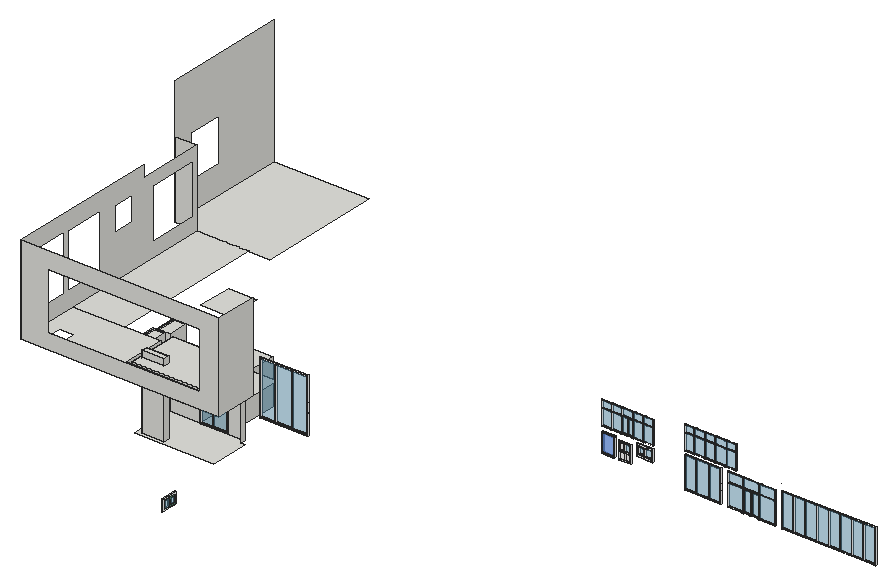
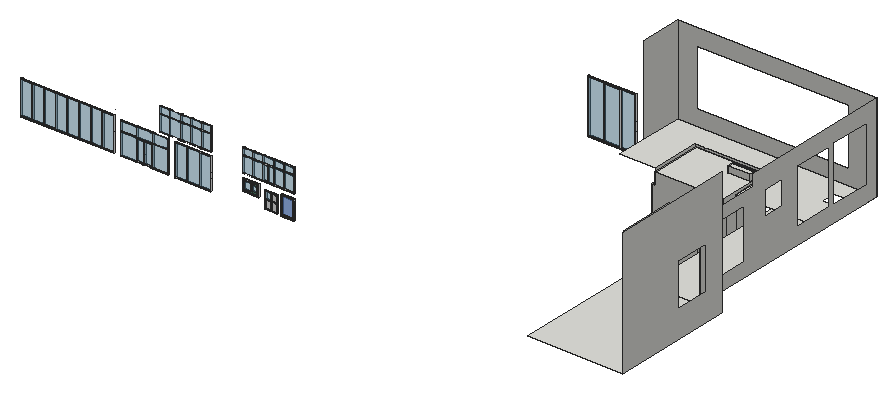
# SketchUp Ruby script. Lengths in inches.
U = 1.inch
M = Sketchup.active_model
def pt(a) = Geom::Point3d.new(a.map { |v| v * U })
def face(e, loops, mat)
  f = e.add_face(loops[0].map { |a| pt(a) })
  loops[1..].each { |l| e.add_face(l.map { |a| pt(a) }).erase! }
  f.material = f.back_material = mat if mat
  f
end
# faces: each face lists its corners as indices into pts; further lists are holes
def faces(e, pts, list, mat = nil) = list.each { |f| face(e, (f[0].is_a?(Array) ? f : [f]).map { |l| l.map { |i| pts[i] } }, mat) }
# xy, xz, yz: faces in a plane at the given z, y or x. An outline is a flat list of corners, or four numbers for a rectangle; further outlines are holes
def ring(l) = l.size == 4 ? [[l[0], l[1]], [l[2], l[1]], [l[2], l[3]], [l[0], l[3]]] : l.each_slice(2).to_a
def flat(e, list, mat, &to3) = list.each { |f| face(e, (f[0].is_a?(Array) ? f : [f]).map { |l| ring(l).map { |u, v| to3.(u, v) } }, mat) }
def xy(e, z, list, mat = nil) = flat(e, list, mat) { |x, y| [x, y, z] }
def xz(e, y, list, mat = nil) = flat(e, list, mat) { |x, z| [x, y, z] }
def yz(e, x, list, mat = nil) = flat(e, list, mat) { |y, z| [x, y, z] }
def lines(e, pts, list) = list.each { |a, b| e.add_line(pt(pts[a]), pt(pts[b])) }
# prism: a flat outline (further loops are holes) pulled along v
def prism(e, loops, v, mat = nil)
  f = face(e, loops, mat); d = Geom::Vector3d.new(v.map { |x| x * U })
  f.pushpull(f.normal.samedirection?(d) ? d.length : -d.length)
end
def box(e, o, s, mat = nil) = prism(e, [[o, [o[0] + s[0], o[1], o[2]], [o[0] + s[0], o[1] + s[1], o[2]], [o[0], o[1] + s[1], o[2]]]], [0, 0, s[2]], mat)
def at(x, y, z, deg = 0) = Geom::Transformation.translation(pt([x, y, z])) * Geom::Transformation.rotation(ORIGIN, Z_AXIS, deg.degrees)
def axes(o, x, y, z) = Geom::Transformation.new([*x, 0, *y, 0, *z, 0, *pt(o).to_a, 1])
def part(name) = M.definitions.add(name)
# library, detail: a bought-in or finely detailed component or shape, given as its bounding box
def library(name, o, s) = part(name).tap { |d| box(d.entities, o, s) }
def detail(e, o, s) = box(e.add_group.entities, o, s)
def put(e, d, t, mat = nil) = e.add_instance(d, t).tap { |i| i.material = mat if mat }
def group(e, t, mat = nil) = e.add_group.tap { |g| g.transformation = t; g.material = mat if mat }.entities
root = M.entities
M.materials.add("Translucent_Glass_Blue1").color = [100, 149, 237]
M.materials["Translucent_Glass_Blue1"].alpha = 0.5
M.materials.add("[0010_Snow]").color = [255, 250, 250]
M.materials.add("[Color_000]").color = [255, 255, 255]
M.materials.add("[Jade]").color = [77, 143, 110]
M.materials.add("[Translucent_Glass_Blue]").color = [100, 149, 237]
M.materials["[Translucent_Glass_Blue]"].alpha = 0.5
M.materials.add("[Translucent_Glass_Blue]1").color = [87, 149, 181]
M.materials["[Translucent_Glass_Blue]1"].alpha = 0.5
c1 = part("Group\#3")
xy(c1.entities,0,[[0,0,2.14,2.21]],"[Color_000]")
xy(c1.entities,1.67,[[2.14,0,29.96,2.21],[29.96,0,32.1,0.88],[32.1,0,64.19,2.21],[64.19,0,66.33,0.88]],"[Color_000]")
xy(c1.entities,84.95,[[2.14,0,29.96,2.21],[29.96,0,32.1,0.88],[32.1,0,64.19,2.21],[64.19,0,66.33,0.88]],"[Color_000]")
xy(c1.entities,86.61,[[0,0,66.33,2.21]],"[Color_000]")
xz(c1.entities,0,[[0,0,0,86.61,66.33,86.61,66.33,84.95,2.14,84.95,2.14,0],[2.14,0,66.33,1.67]],"[Color_000]")
xz(c1.entities,0.88,[[29.96,1.67,32.1,84.95],[64.19,1.67,66.33,84.95]],"[Color_000]")
xz(c1.entities,2.21,[[2.14,1.67,29.96,84.95],[32.1,1.67,64.19,84.95]],"[Translucent_Glass_Blue]1")
yz(c1.entities,0,[[0,0,2.21,32.8125],[0,32.8125,2.21,48.3],[0,48.3,2.21,86.61]],"[Color_000]")
yz(c1.entities,2.14,[[0,1.67,2.21,84.95]],"[Color_000]")
yz(c1.entities,29.96,[[0.88,1.67,2.21,84.95]],"[Color_000]")
yz(c1.entities,32.1,[[0.88,1.67,2.21,84.95]],"[Color_000]")
yz(c1.entities,64.19,[[0.88,1.67,2.21,84.95]],"[Color_000]")
yz(c1.entities,66.33,[[0.88,1.67,2.21,84.95]],"[Color_000]")
c2 = part("ProLine-Casement-Window")
xy(c2.entities,-3.73,[[[0,0,29,59],[0.74,0.74,28.26,58.26]]],"[Color_000]")
xy(c2.entities,-3.07,[[[1.32,1.32,27.68,57.68],[1.72,1.73,27.28,57.375]]],"[Color_000]")
xy(c2.entities,-1.67,[[1.72,2.22,1.875,57.125],[27.125,2.22,27.28,57.125]],"[Color_000]")
xy(c2.entities,-1.14,[[[1.875,2.22,27.125,57.125],[2.38,2.38,26.65,56.69]]],"[Color_000]")
xy(c2.entities,-0.52,[[2.51,2.51,26.52,56.5625]],"Translucent_Glass_Blue1")
xy(c2.entities,-0.52,[[[2.01,2.05,26.99,57.04],[2.51,2.51,26.52,56.5625]]],"[Color_000]")
xy(c2.entities,0.16,[[[2.01,2.05,26.99,57.04],[2.51,2.51,26.52,56.5625]]],"[Color_000]")
xy(c2.entities,0.16,[[2.51,2.51,26.52,56.5625]],"[Translucent_Glass_Blue]")
xy(c2.entities,0.63,[[[0.77,0.77,28.23,58.23],[2.42,2.42,26.61,56.66]]],"[Color_000]")
xy(c2.entities,1.2,[[[0.57,0.57,28.43,58.43],[0.77,0.77,28.23,58.23]]],"[Color_000]")
xy(c2.entities,1.25,[[[0,0,29,59],[0.39,0.39,28.61,58.61]]],"[Color_000]")
xz(c2.entities,0,[[0,-3.73,29,0],[0,0,29,1.25]],"[Color_000]")
xz(c2.entities,0.77,[[0.77,0.63,28.23,1.2]],"[Color_000]")
xz(c2.entities,2.05,[[2.01,-0.52,26.99,0.16]],"[Color_000]")
xz(c2.entities,2.22,[[1.875,-1.67,27.125,-1.14]],"[Color_000]")
xz(c2.entities,57.04,[[2.01,-0.52,26.99,0.16]],"[Color_000]")
xz(c2.entities,57.125,[[1.875,-1.67,27.125,-1.14]],"[Color_000]")
xz(c2.entities,57.375,[[1.72,-3.07,27.28,-2.84]],"[Color_000]")
xz(c2.entities,58.23,[[0.77,0.63,28.23,1.2]],"[Color_000]")
xz(c2.entities,59,[[0,-3.73,29,0],[0,0,29,1.25]],"[Color_000]")
yz(c2.entities,0,[[0,-3.73,59,0],[0,0,59,1.25]],"[Color_000]")
yz(c2.entities,0.77,[[0.77,0.63,58.23,1.2]],"[Color_000]")
yz(c2.entities,1.72,[[1.73,-3.07,57.375,-3.07,57.375,-2.84,57.125,-1.67,2.22,-1.67,1.96,-2.89]],"[Color_000]")
yz(c2.entities,1.875,[[2.22,-1.67,57.125,-1.14]],"[Color_000]")
yz(c2.entities,2.01,[[2.05,-0.52,57.04,0.16]],"[Color_000]")
yz(c2.entities,26.99,[[2.05,-0.52,57.04,0.16]],"[Color_000]")
yz(c2.entities,27.125,[[2.22,-1.67,57.125,-1.14]],"[Color_000]")
yz(c2.entities,27.28,[[1.73,-3.07,1.96,-2.89,2.22,-1.67,57.125,-1.67,57.375,-2.84,57.375,-3.07]],"[Color_000]")
yz(c2.entities,28.23,[[0.77,0.63,58.23,1.2]],"[Color_000]")
yz(c2.entities,29,[[0,-3.73,59,0],[0,0,59,1.25]],"[Color_000]")
p = [[0.74,58.26,-3.73],[1.32,57.68,-3.07],[1.32,57.375,-3.07],[1.32,1.73,-3.07],[1.32,1.32,-3.07],[0.74,0.74,-3.73],
  [27.68,1.32,-3.07],[28.26,0.74,-3.73],[27.68,57.68,-3.07],[28.26,58.26,-3.73],[27.68,1.73,-3.07],[27.68,57.375,-3.07],
  [27.28,1.73,-3.07],[1.72,1.73,-3.07],[1.72,1.96,-2.89],[27.28,1.96,-2.89],[1.72,2.22,-1.67],[1.875,2.22,-1.67],
  [27.125,2.22,-1.67],[27.28,2.22,-1.67],[27.125,57.125,-1.67],[1.875,57.125,-1.67],[1.72,57.125,-1.67],[1.72,57.375,-2.84],
  [27.28,57.375,-2.84],[27.28,57.125,-1.67],[2.51,56.5625,-0.52],[2.51,2.51,-0.52],[2.38,2.38,-1.14],[2.38,56.69,-1.14],
  [26.65,2.38,-1.14],[2.77,2.51,-0.52],[26.14,2.51,-0.52],[26.52,2.51,-0.52],[26.52,56.5625,-0.52],[26.65,56.69,-1.14],
  [2.51,2.51,0.16],[2.51,56.5625,0.16],[2.42,56.66,0.63],[2.42,2.42,0.63],[26.52,2.51,0.16],[26.14,2.51,0.16],
  [2.77,2.51,0.16],[26.61,2.42,0.63],[26.52,56.5625,0.16],[26.61,56.66,0.63],[0.57,0.57,1.2],[0.57,58.43,1.2],
  [0.39,58.61,1.25],[0.39,0.39,1.25],[28.43,0.57,1.2],[28.61,0.39,1.25],[28.43,58.43,1.2],[28.61,58.61,1.25],
  [0.75,58.43,1.2],[0.77,58.43,1.2],[28.23,58.43,1.2],[28.25,58.43,1.2]]
faces(c2.entities,p,[[0,1,2,3,4,5],[5,4,6,7],[8,9,7,6,10,11],[1,0,9,8],[12,13,14,15],[16,17,18,19,15,14],[20,21,22,23,24,25],[26,27,28,29],
  [30,28,27,31,32,33],[33,34,35,30],[34,26,29,35],[36,37,38,39],[40,41,42,36,39,43],[44,40,43,45],[38,37,44,45],[46,47,48,49],
  [50,46,49,51],[52,50,51,53],[53,48,47,54,55,56,57,52]],"[Color_000]")
c3 = part("Group\#65")
xy(c3.entities,0,[[[275.59,275.59,3818.9,2244.09],[393.7,393.7,1909.45,2125.98],[2381.89,590.55,3503.9375,1929.13]]])
xy(c3.entities,0,[[[0,0,4094.49,2519.69],[275.59,275.59,3818.9,2244.09]]],"[Color_000]")
xy(c3.entities,0,[[393.7,393.7,1909.45,2125.98],[2381.89,590.55,3503.9375,1929.13]],"[Translucent_Glass_Blue]1")
xy(c3.entities,157.48,[[[2106.3,314.96,3779.53,2204.72],[2381.89,590.55,3503.9375,1929.13]]],"[Color_000]")
xy(c3.entities,196.85,[[[275.59,275.59,3818.9,2244.09],[2106.3,314.96,3779.53,2204.72],[393.7,393.7,1909.45,2125.98]]],"[Color_000]")
xy(c3.entities,236.22,[[[0,0,4094.49,2519.69],[275.59,275.59,3818.9,2244.09]]],"[Color_000]")
xz(c3.entities,0,[[0,0,4094.49,236.22]],"[Color_000]")
xz(c3.entities,275.59,[[275.59,0,3818.9,196.85],[275.59,196.85,3818.9,236.22]],"[Color_000]")
xz(c3.entities,314.96,[[2106.3,157.48,3779.53,196.85]],"[Color_000]")
xz(c3.entities,393.7,[[393.7,0,1909.45,196.85]],"[Color_000]")
xz(c3.entities,590.55,[[2381.89,0,3503.9375,157.48]],"[Color_000]")
xz(c3.entities,1929.13,[[2381.89,0,3503.9375,157.48]],"[Color_000]")
xz(c3.entities,2125.98,[[393.7,0,1909.45,196.85]],"[Color_000]")
xz(c3.entities,2204.72,[[2106.3,157.48,3779.53,196.85]],"[Color_000]")
xz(c3.entities,2244.09,[[275.59,0,3818.9,196.85],[275.59,196.85,3818.9,236.22]],"[Color_000]")
xz(c3.entities,2519.69,[[0,0,4094.49,236.22]],"[Color_000]")
yz(c3.entities,0,[[0,0,2519.69,236.22]],"[Color_000]")
yz(c3.entities,275.59,[[275.59,0,2244.09,196.85],[275.59,196.85,2244.09,236.22]],"[Color_000]")
yz(c3.entities,393.7,[[393.7,0,2125.98,196.85]],"[Color_000]")
yz(c3.entities,1909.45,[[393.7,0,2125.98,196.85]],"[Color_000]")
yz(c3.entities,2106.3,[[314.96,157.48,2204.72,196.85]],"[Color_000]")
yz(c3.entities,2381.89,[[590.55,0,1929.13,157.48]],"[Color_000]")
yz(c3.entities,3503.9375,[[590.55,0,1929.13,157.48]],"[Color_000]")
yz(c3.entities,3779.53,[[314.96,157.48,2204.72,196.85]],"[Color_000]")
yz(c3.entities,3818.9,[[275.59,0,2244.09,196.85],[275.59,196.85,2244.09,236.22]],"[Color_000]")
yz(c3.entities,4094.49,[[0,0,2519.69,236.22]],"[Color_000]")
c4 = part("Group\#66")
xy(c4.entities,0,[[8858.27,0,9055.12,10236.22]],"[Color_000]")
xy(c4.entities,0,[[196.85,196.85,2755.91,10039.37],[2952.76,196.85,5905.51,10039.37],[6102.36,196.85,8858.27,10039.37]],"[Translucent_Glass_Blue]1")
xy(c4.entities,118.11,[[2755.91,196.85,2952.76,10039.37],[5905.51,196.85,6102.36,10039.37]],"[Color_000]")
xy(c4.entities,196.85,[[0,0,0,10236.22,8858.27,10236.22,8858.27,10039.37,196.85,10039.37,196.85,0],[196.85,0,8858.27,196.85],[8858.27,0,9055.12,10236.22]],"[Color_000]")
xz(c4.entities,0,[[0,0,196.85,196.85],[196.85,0,8858.27,196.85],[8858.27,0,9055.12,196.85]],"[Color_000]")
xz(c4.entities,196.85,[[196.85,0,2755.91,196.85],[2952.76,0,5905.51,196.85],[6102.36,0,8858.27,196.85],[2755.91,118.11,2952.76,196.85],[5905.51,118.11,6102.36,196.85]],"[Color_000]")
xz(c4.entities,10039.37,[[196.85,0,2755.91,196.85],[2952.76,0,5905.51,196.85],[6102.36,0,8858.27,196.85],[2755.91,118.11,2952.76,196.85],[5905.51,118.11,6102.36,196.85]],"[Color_000]")
xz(c4.entities,10236.22,[[0,0,8858.27,196.85],[8858.27,0,9055.12,196.85]],"[Color_000]")
yz(c4.entities,0,[[0,0,3877.95,196.85],[3877.95,0,5708.66,196.85],[5708.66,0,10236.22,196.85]],"[Color_000]")
yz(c4.entities,196.85,[[196.85,0,10039.37,196.85]],"[Color_000]")
yz(c4.entities,2755.91,[[196.85,0,10039.37,118.11]],"[Color_000]")
yz(c4.entities,2952.76,[[196.85,0,10039.37,118.11]],"[Color_000]")
yz(c4.entities,5905.51,[[196.85,0,10039.37,118.11]],"[Color_000]")
yz(c4.entities,6102.36,[[196.85,0,10039.37,118.11]],"[Color_000]")
yz(c4.entities,8858.27,[[0,0,196.85,196.85],[196.85,0,10039.37,196.85]],"[Color_000]")
yz(c4.entities,9055.12,[[0,0,3877.95,196.85],[3877.95,0,5708.66,196.85],[5708.66,0,10236.22,196.85]],"[Color_000]")
xy(root,54.6875,[[[298.73,288.02,514.54,288.02,514.54,394.71,502.61,394.71,502.61,409.08,455.75,409.08,455.75,562.14,380.43,562.14,380.43,409.08,298.73,409.08],[310.99,299.24,370.42,314.05]]])
xy(root,134.84,[[200.3125,488.22,237.4375,540.72]])
xy(root,142.375,[[200.3125,420.82,232.8125,472.44]])
xy(root,176.55,[[380.43,409.08,455.75,562.14]])
xy(root,177.99,[[200.3125,638.47,277.875,731.65]])
xy(root,187.34,[[200.3125,488.22,237.4375,540.72]])
xy(root,194,[[200.3125,420.82,232.8125,472.44]])
xy(root,207.625,[[298.73,260.71,298.73,409.08,306.54,409.08,306.54,269.58,492.91,269.58,492.91,409.08,502.61,409.08,502.61,260.71]])
xy(root,240,[[[60,198.52,60,378.52,298.73,378.52,298.73,260.71,502.61,260.71,502.61,394.71,600,394.71,600,198.52],[98.56,244.91,139.12,285.48]],[306.54,269.58,492.91,409.08],[60,378.52,200.3125,798.52],[0,798.52,258.9375,1134.21]])
xy(root,256.3125,[[310.99,299.24,370.42,314.05]])
xz(root,198.52,[[[60,240,600,480],[134.85,281.62,547.79,436.43]]])
xz(root,260.71,[[298.73,207.625,502.61,240]])
xz(root,269.58,[[306.54,207.625,492.91,240]])
xz(root,299.24,[[310.99,54.6875,370.42,256.3125]])
xz(root,314.05,[[310.99,54.6875,370.42,256.3125]])
xz(root,409.08,[[298.73,54.6875,380.43,54.6875,380.43,176.55,455.75,176.55,455.75,54.6875,502.61,54.6875,502.61,207.625,492.91,207.625,492.91,240,306.54,240,306.54,207.625,298.73,207.625]])
xz(root,420.82,[[200.3125,142.375,232.8125,194]])
xz(root,472.44,[[200.3125,142.375,232.8125,194]])
xz(root,488.22,[[200.3125,134.84,237.4375,187.34]])
xz(root,540.72,[[200.3125,134.84,237.4375,187.34]])
xz(root,562.14,[[380.43,54.6875,455.75,176.55]])
xz(root,798.52,[[0,240,60,448.41]])
yz(root,0,[[[798.52,240,1134.21,584.21],[852.4375,316.09,949.6875,433.4]]])
yz(root,60,[[[198.52,240,198.52,480,618.52,480,618.52,448.41,798.52,448.41,798.52,240],[649.71,278.09,786.4,414.78],[232.46,283.68,347.46,434.87],[360.8,284.7,469.11,432.07],[520.01,358.15,578.58,423.47]]])
yz(root,232.8125,[[420.82,142.375,472.44,194]])
yz(root,237.4375,[[488.22,134.84,540.72,187.34]])
yz(root,298.73,[[378.52,54.6875,409.08,207.625],[260.71,207.625,378.52,240]])
yz(root,306.54,[[269.58,207.625,409.08,240]])
yz(root,310.99,[[299.24,54.6875,314.05,256.3125]])
yz(root,370.42,[[299.24,54.6875,314.05,256.3125]])
yz(root,380.43,[[409.08,54.6875,562.14,176.55]])
yz(root,455.75,[[409.08,54.6875,562.14,176.55]])
yz(root,492.91,[[269.58,207.625,409.08,240]])
yz(root,502.61,[[394.71,54.6875,409.08,207.625],[260.71,207.625,394.71,240]])
yz(root,600,[[198.52,240,313.58,480]])
put(root,c1,axes([380.43,409.08,54.6875],[1.13542,0,0],[0,1,0],[0,0,1.41]))
g1 = group(root,at(1639.67,815.55,62.11),"[Jade]")
xy(g1,0,[[0,-1.77,1.77,0],[1.77,-1.77,253.35,0],[253.35,-1.77,255.12,0]],"[Color_000]")
xy(g1,1.77,[[1.77,-1.77,30.41,0],[32.19,-1.77,61.71,0],[63.48,-1.77,93.9,0],[95.67,-1.77,126.08,0],[127.85,-1.77,157.68,0],
  [159.45,-1.77,189.27,0],[191.04,-1.77,220.87,0],[222.64,-1.77,253.35,0]],"[Color_000]")
xy(g1,90.35,[[1.77,-1.77,30.41,0],[32.19,-1.77,61.71,0],[63.48,-1.77,93.9,0],[95.67,-1.77,126.08,0],[127.85,-1.77,157.68,0],
  [159.45,-1.77,189.27,0],[191.04,-1.77,220.87,0],[222.64,-1.77,253.35,0]],"[Color_000]")
xy(g1,92.125,[[0,-1.77,255.12,0]],"[Color_000]")
xz(g1,-1.77,[[0,0,0,92.125,255.12,92.125,255.12,0,253.35,0,253.35,90.35,1.77,90.35,1.77,0],[1.77,0,253.35,1.77],[30.41,1.77,32.19,90.35],[61.71,1.77,63.48,90.35],[93.9,1.77,95.67,90.35],
  [126.08,1.77,127.85,90.35],[157.68,1.77,159.45,90.35],[189.27,1.77,191.04,90.35],[220.87,1.77,222.64,90.35]],"[Color_000]")
xz(g1,0,[[1.77,1.77,30.41,90.35],[32.19,1.77,61.71,90.35],[63.48,1.77,93.9,90.35],[95.67,1.77,126.08,90.35],[127.85,1.77,157.68,90.35],
  [159.45,1.77,189.27,90.35],[191.04,1.77,220.87,90.35],[222.64,1.77,253.35,90.35]],"[Translucent_Glass_Blue]1")
yz(g1,0,[[-1.77,0,0,51.38],[-1.77,51.38,0,92.125]],"[Color_000]")
yz(g1,1.77,[[-1.77,1.77,0,90.35]],"[Color_000]")
yz(g1,30.41,[[-1.77,1.77,0,90.35]],"[Color_000]")
yz(g1,32.19,[[-1.77,1.77,0,90.35]],"[Color_000]")
yz(g1,61.71,[[-1.77,1.77,0,90.35]],"[Color_000]")
yz(g1,63.48,[[-1.77,1.77,0,90.35]],"[Color_000]")
yz(g1,93.9,[[-1.77,1.77,0,90.35]],"[Color_000]")
yz(g1,95.67,[[-1.77,1.77,0,90.35]],"[Color_000]")
yz(g1,126.08,[[-1.77,1.77,0,90.35]],"[Color_000]")
yz(g1,127.85,[[-1.77,1.77,0,90.35]],"[Color_000]")
yz(g1,157.68,[[-1.77,1.77,0,90.35]],"[Color_000]")
yz(g1,159.45,[[-1.77,1.77,0,90.35]],"[Color_000]")
yz(g1,189.27,[[-1.77,1.77,0,90.35]],"[Color_000]")
yz(g1,191.04,[[-1.77,1.77,0,90.35]],"[Color_000]")
yz(g1,220.87,[[-1.77,1.77,0,90.35]],"[Color_000]")
yz(g1,222.64,[[-1.77,1.77,0,90.35]],"[Color_000]")
yz(g1,253.35,[[-1.77,1.77,0,90.35]],"[Color_000]")
yz(g1,255.12,[[-1.77,0,0,92.125]],"[Color_000]")
g2 = group(root,at(1490.58,816.74,62.11),"[Color_000]")
xy(g2,86.93,[[129.04,-2.17,130.39,0],[87.61,-1.36,129.04,0]])
xz(g2,-2.17,[[129.04,0,130.39,86.93]])
xz(g2,-1.36,[[87.61,85.57,129.04,86.93]])
xz(g2,0,[[129.04,0,130.39,86.93],[87.61,85.57,129.04,86.93]])
yz(g2,129.04,[[-2.17,85.57,-1.36,86.93],[-1.36,85.57,0,86.93]])
yz(g2,130.39,[[-2.17,0,0,86.93]])
p = [[144.66,0,107.3],[144.66,0,108.66]]
lines(g2,p,[[0,1]])
g3 = group(g2,at(0,0,0),"[Color_000]")
xy(g3,0,[[0,-2.17,1.36,0],[42.79,-2.17,44.14,0],[86.25,-2.17,87.61,0],[129.04,-2.17,130.39,0],[1.36,-1.36,42.79,0],
  [44.14,-1.36,86.25,0],[87.61,-1.36,129.04,0]])
xy(g3,1.36,[[1.36,-1.36,42.79,0],[44.14,-1.36,65.18,-0.81],[65.18,-1.36,65.22,0],[65.22,-1.36,86.25,-0.81],[87.61,-1.36,129.04,0]])
xy(g3,2.91,[[45.7,-0.81,63.62,0],[66.77,-0.81,84.7,0]])
xy(g3,57.53,[[45.7,-0.81,63.62,0],[66.77,-0.81,84.7,0]])
xy(g3,59.08,[[1.36,-1.36,42.79,0],[44.14,-1.36,65.18,-0.81],[65.18,-1.36,65.22,0],[65.22,-1.36,86.25,-0.81],[87.61,-1.36,129.04,0]])
xy(g3,60.44,[[1.36,-1.36,42.79,0],[44.14,-1.36,86.25,0],[87.61,-1.36,129.04,0]])
xy(g3,85.57,[[1.36,-1.36,42.79,0],[44.14,-1.36,86.25,0],[87.61,-1.36,129.04,0]])
xy(g3,86.93,[[0,-2.17,1.36,0],[42.79,-2.17,44.14,0],[86.25,-2.17,87.61,0],[1.36,-1.36,42.79,0],[44.14,-1.36,86.25,0]])
xz(g3,-2.17,[[0,0,1.36,86.93],[42.79,0,44.14,86.93],[86.25,0,87.61,86.93]])
xz(g3,-1.36,[[1.36,0,42.79,1.36],[44.14,0,86.25,1.36],[87.61,0,129.04,1.36],[1.36,59.08,42.79,60.44],[44.14,59.08,86.25,60.44],
  [87.61,59.08,129.04,60.44],[1.36,85.57,42.79,86.93],[44.14,85.57,86.25,86.93]])
xz(g3,-0.81,[[[44.14,1.36,65.18,59.08],[45.7,2.91,63.62,57.53]],[[65.22,1.36,86.25,59.08],[66.77,2.91,84.7,57.53]]])
xz(g3,0,[[65.18,1.36,65.22,59.08]])
xz(g3,0,[[1.36,1.36,42.79,59.08],[87.61,1.36,129.04,59.08],[45.7,2.91,63.62,57.53],[66.77,2.91,84.7,57.53],[1.36,60.44,42.79,85.57],
  [44.14,60.44,86.25,85.57],[87.61,60.44,129.04,85.57]],"[Translucent_Glass_Blue]1")
yz(g3,0,[[-2.17,0,0,86.93]])
yz(g3,1.36,[[-2.17,0,-1.36,1.36],[-2.17,1.36,0,59.08],[-2.17,59.08,-1.36,60.44],[-2.17,60.44,0,85.57],[-2.17,85.57,-1.36,86.93]])
yz(g3,42.79,[[-2.17,0,-1.36,1.36],[-2.17,1.36,0,59.08],[-2.17,59.08,-1.36,60.44],[-2.17,60.44,0,85.57],[-2.17,85.57,-1.36,86.93]])
yz(g3,44.14,[[-2.17,0,-1.36,1.36],[-2.17,1.36,-0.81,59.08],[-2.17,59.08,-1.36,60.44],[-2.17,60.44,0,85.57],[-2.17,85.57,-1.36,86.93]])
yz(g3,45.7,[[-0.81,2.91,0,57.53]])
yz(g3,63.62,[[-0.81,2.91,0,28.27],[-0.81,28.27,0,57.53]])
yz(g3,65.18,[[-0.81,1.36,0,59.08]])
yz(g3,65.22,[[-0.81,1.36,0,59.08]])
yz(g3,66.77,[[-0.81,2.91,0,28.27],[-0.81,28.27,0,57.53]])
yz(g3,84.7,[[-0.81,2.91,0,57.53]])
yz(g3,86.25,[[-2.17,0,-1.36,1.36],[-2.17,1.36,-0.81,59.08],[-2.17,59.08,-1.36,60.44],[-2.17,60.44,0,85.57],[-2.17,85.57,-1.36,86.93]])
yz(g3,87.61,[[-2.17,0,-1.36,1.36],[-2.17,1.36,0,59.08],[-2.17,59.08,-1.36,60.44],[-2.17,60.44,0,85.57],[-2.17,85.57,-1.36,86.93]])
yz(g3,129.04,[[-2.17,0,-1.36,1.36],[-1.36,0,0,1.36],[-2.17,1.36,0,59.08],[-2.17,59.08,-1.36,60.44],[-1.36,59.08,0,60.44],
  [-2.17,60.44,0,85.57]])
p = [[87.61,0,85.57],[87.61,0,86.93]]
lines(g3,p,[[0,1]])
g4 = group(root,at(1373.45,817.96,62.11),"[Jade]")
xy(g4,0,[[0,-2.21,2.14,0],[2.14,-2.21,96.29,0],[96.29,-2.21,98.43,0]],"[Color_000]")
xy(g4,1.67,[[2.14,-2.21,29.96,0],[29.96,-2.21,32.1,-1.32],[32.1,-2.21,64.19,0],[64.19,-2.21,66.33,-1.32],[66.33,-2.21,96.29,0]],"[Color_000]")
xy(g4,84.95,[[2.14,-2.21,29.96,0],[29.96,-2.21,32.1,-1.32],[32.1,-2.21,64.19,0],[64.19,-2.21,66.33,-1.32],[66.33,-2.21,96.29,0]],"[Color_000]")
xy(g4,86.61,[[0,-2.21,96.29,0],[96.29,-2.21,98.43,0]],"[Color_000]")
xz(g4,-2.21,[[0,0,0,86.61,96.29,86.61,96.29,84.95,2.14,84.95,2.14,0],[2.14,0,96.29,1.67],[96.29,0,98.43,86.61]],"[Color_000]")
xz(g4,-1.32,[[29.96,1.67,32.1,84.95],[64.19,1.67,66.33,84.95]],"[Color_000]")
xz(g4,0,[[96.29,0,98.43,86.61]],"[Color_000]")
xz(g4,0,[[2.14,1.67,29.96,84.95],[32.1,1.67,64.19,84.95],[66.33,1.67,96.29,84.95]],"[Translucent_Glass_Blue]1")
yz(g4,0,[[-2.21,0,0,32.8125],[-2.21,32.8125,0,48.3],[-2.21,48.3,0,86.61]],"[Color_000]")
yz(g4,2.14,[[-2.21,1.67,0,84.95]],"[Color_000]")
yz(g4,29.96,[[-1.32,1.67,0,84.95]],"[Color_000]")
yz(g4,32.1,[[-1.32,1.67,0,84.95]],"[Color_000]")
yz(g4,64.19,[[-1.32,1.67,0,84.95]],"[Color_000]")
yz(g4,66.33,[[-1.32,1.67,0,84.95]],"[Color_000]")
yz(g4,96.29,[[-2.21,0,0,1.67],[-2.21,1.67,0,84.95]],"[Color_000]")
yz(g4,98.43,[[-2.21,0,0,32.8125],[-2.21,32.8125,0,48.3],[-2.21,48.3,0,86.61]],"[Color_000]")
put(root,c2,axes([1181.72,818.09,123.22],[-1.22183,0,0],[0,0,-0.86733],[0,-0.94586,0]),"[0010_Snow]")
g5 = group(root,at(1192.27,818.48,72.39),"[Color_000]")
xy(g5,0,[[0,-1.57,34.25,0]],"[Color_000]")
xy(g5,1.97,[[17.81,-1.57,32.28,0]])
xy(g5,1.97,[[1.97,-1.57,16.4375,0]],"[Color_000]")
xy(g5,22.34,[[1.97,-1.57,16.4375,0]])
xy(g5,22.34,[[17.81,-1.57,32.28,0]],"[Color_000]")
xy(g5,23.33,[[1.57,-1.57,16.83,-0.98],[1.57,-0.98,16.83,0]])
xy(g5,23.72,[[17.81,-1.57,32.28,0]])
xy(g5,24.7,[[2.95,-0.98,15.45,0]],"[Color_000]")
xy(g5,43.11,[[2.95,-0.98,15.45,0]],"[Color_000]")
xy(g5,44.09,[[17.81,-1.57,32.28,0]],"[Color_000]")
xy(g5,44.49,[[1.57,-1.57,2.23,-0.98],[2.23,-1.57,16.83,-0.98],[1.57,-0.98,2.23,0],[2.23,-0.98,16.83,0]])
xy(g5,46.0625,[[0,-1.57,34.25,0]])
xz(g5,-1.57,[[[0,0,34.25,46.0625],[1.57,23.33,16.83,44.49],[1.97,1.97,16.4375,22.34],[17.81,1.97,32.28,22.34],[17.81,23.72,32.28,44.09]]],"[Color_000]")
xz(g5,-0.98,[[[1.57,23.33,16.83,44.49],[2.95,24.7,15.45,43.11]]],"[Color_000]")
xz(g5,0,[[[0,0,34.25,46.0625],[1.57,23.33,16.83,44.49],[1.97,1.97,16.4375,22.34],[17.81,1.97,32.28,22.34],[17.81,23.72,32.28,44.09]],[1.97,1.97,16.4375,22.34],[17.81,1.97,32.28,22.34],[[1.57,23.33,16.83,44.49],[2.95,24.7,15.45,43.11]],[2.95,24.7,15.45,43.11]],"[Color_000]")
xz(g5,0,[[17.81,23.72,32.28,44.09]],"[Translucent_Glass_Blue]1")
yz(g5,0,[[-1.57,0,0,46.0625]])
yz(g5,1.57,[[-1.57,23.33,-0.98,44.49],[-0.98,23.33,0,44.49]])
yz(g5,1.97,[[-1.57,1.97,0,22.34]])
yz(g5,2.95,[[-0.98,24.7,0,43.11]],"[Color_000]")
yz(g5,15.45,[[-0.98,24.7,0,43.11]],"[Color_000]")
yz(g5,16.4375,[[-1.57,1.97,0,22.34]])
yz(g5,16.83,[[-1.57,23.33,-0.98,44.49],[-0.98,23.33,0,44.49]])
yz(g5,17.81,[[-1.57,1.97,0,22.34],[-1.57,23.72,0,44.09]])
yz(g5,32.28,[[-1.57,23.72,0,44.09]])
yz(g5,32.28,[[-1.57,1.97,0,22.34]],"[Color_000]")
yz(g5,34.25,[[-1.57,0,0,46.0625]],"[Color_000]")
put(root,c3,axes([1284.32,821.73,128.22],[-0.01082,0,0],[0,0,-0.0125],[0,-0.01406,0]),"[Jade]")
put(root,c3,axes([607.59,0,128.22],[0,0.01082,0],[0,0,-0.0125],[-0.01406,0,0]),"[Jade]")
put(root,c3,axes([205.82,488.22,187.125],[0,0.01282,0],[0,0,-0.02075],[-0.02333,0,0]),"[Jade]")
g6 = group(root,at(1146.29,818.94,137.79),"[Color_000]")
xy(g6,0,[[0,-2.04,0.98,0],[27.3125,-2.04,28.3,0],[54.625,-2.04,55.61,0],[86.12,-2.04,87.11,0],[113.44,-2.04,114.42,0],
  [140.75,-2.04,141.73,0],[0.98,-1.27,27.3125,0],[28.3,-1.27,54.625,0],[55.61,-1.27,86.12,0],[87.11,-1.27,113.44,0],
  [114.42,-1.27,140.75,0]],"[Color_000]")
xy(g6,1,[[0.98,-1.27,27.3125,0],[28.3,-1.27,54.625,0],[55.61,-1.27,70.85,-0.76],[70.85,-1.27,70.88,-0.76],[70.88,-1.27,86.12,-0.76],
  [87.11,-1.27,113.44,0],[114.42,-1.27,140.75,0]],"[Color_000]")
xy(g6,2.14,[[56.74,-0.76,69.73,0],[72.01,-0.76,85,0]],"[Color_000]")
xy(g6,42.34,[[56.74,-0.76,69.73,0],[72.01,-0.76,85,0]],"[Color_000]")
xy(g6,43.48,[[0.98,-1.27,27.3125,0],[28.3,-1.27,54.625,0],[55.61,-1.27,70.85,-0.76],[70.85,-1.27,70.88,-0.76],[70.88,-1.27,86.12,-0.76],
  [87.11,-1.27,113.44,0],[114.42,-1.27,140.75,0]],"[Color_000]")
xy(g6,44.48,[[0.98,-1.27,27.3125,0],[28.3,-1.27,54.625,0],[55.61,-1.27,86.12,0],[87.11,-1.27,113.44,0],[114.42,-1.27,140.75,0]],"[Color_000]")
xy(g6,62.98,[[0.98,-1.27,27.3125,0],[28.3,-1.27,54.625,0],[55.61,-1.27,86.12,0],[87.11,-1.27,113.44,0],[114.42,-1.27,140.75,0]],"[Color_000]")
xy(g6,63.98,[[0,-2.04,0.98,0],[27.3125,-2.04,28.3,0],[54.625,-2.04,55.61,0],[86.12,-2.04,87.11,0],[113.44,-2.04,114.42,0],
  [140.75,-2.04,141.73,0],[0.98,-1.27,27.3125,0],[28.3,-1.27,54.625,0],[55.61,-1.27,86.12,0],[87.11,-1.27,113.44,0],
  [114.42,-1.27,140.75,0]],"[Color_000]")
xz(g6,-2.04,[[0,0,0.98,63.98],[27.3125,0,28.3,63.98],[54.625,0,55.61,63.98],[86.12,0,87.11,63.98],[113.44,0,114.42,63.98],
  [140.75,0,141.73,63.98]],"[Color_000]")
xz(g6,-1.27,[[0.98,0,27.3125,1],[28.3,0,54.625,1],[55.61,0,86.12,1],[87.11,0,113.44,1],[114.42,0,140.75,1],
  [0.98,43.48,27.3125,44.48],[28.3,43.48,54.625,44.48],[55.61,43.48,86.12,44.48],[87.11,43.48,113.44,44.48],[114.42,43.48,140.75,44.48],
  [0.98,62.98,27.3125,63.98],[28.3,62.98,54.625,63.98],[55.61,62.98,86.12,63.98],[87.11,62.98,113.44,63.98],[114.42,62.98,140.75,63.98]],"[Color_000]")
xz(g6,-0.76,[[[55.61,1,70.85,43.48],[56.74,2.14,69.73,42.34]],[[70.85,1,86.12,43.48],[72.01,2.14,85,42.34]]],"[Color_000]")
xz(g6,0,[[[0,0,0,63.98,140.75,63.98,140.75,62.98,114.42,62.98,114.42,44.48,140.75,44.48,140.75,43.48,114.42,43.48,114.42,1,140.75,1,140.75,0],[87.11,1,113.44,43.48],[0.98,1,27.3125,43.48],[28.3,1,54.625,43.48],[55.61,44.48,86.12,62.98],[72.01,2.14,85,42.34],[56.74,2.14,69.73,42.34],[87.11,44.48,113.44,62.98],[28.3,44.48,54.625,62.98],[0.98,44.48,27.3125,62.98]]])
xz(g6,0,[[140.75,0,141.73,63.98]],"[Color_000]")
xz(g6,0,[[0.98,1,27.3125,43.48],[28.3,1,54.625,43.48],[87.11,1,113.44,43.48],[114.42,1,140.75,43.48],[56.74,2.14,69.73,42.34],
  [72.01,2.14,85,42.34],[0.98,44.48,27.3125,62.98],[28.3,44.48,54.625,62.98],[55.61,44.48,86.12,62.98],[87.11,44.48,113.44,62.98],
  [114.42,44.48,140.75,62.98]],"[Translucent_Glass_Blue]1")
yz(g6,0,[[-2.04,0,0,63.98]],"[Color_000]")
yz(g6,0.98,[[-2.04,0,-1.27,1],[-2.04,1,0,43.48],[-2.04,43.48,-1.27,43.98],[-2.04,43.98,-1.27,44.48],[-2.04,44.48,0,62.98],
  [-2.04,62.98,-1.27,63.98]],"[Color_000]")
yz(g6,27.3125,[[-2.04,0,-1.27,1],[-2.04,1,0,43.48],[-2.04,43.48,-1.27,43.98],[-2.04,43.98,-1.27,44.48],[-2.04,44.48,0,62.98],
  [-2.04,62.98,-1.27,63.98]],"[Color_000]")
yz(g6,28.3,[[-2.04,0,-1.27,1],[-2.04,1,0,43.48],[-2.04,43.48,-1.27,43.98],[-2.04,43.98,-1.27,44.48],[-2.04,44.48,0,62.98],
  [-2.04,62.98,-1.27,63.98]],"[Color_000]")
yz(g6,54.625,[[-2.04,0,-1.27,1],[-2.04,1,0,43.48],[-2.04,43.48,-1.27,43.98],[-2.04,43.98,-1.27,44.48],[-2.04,44.48,0,62.98],
  [-2.04,62.98,-1.27,63.98]],"[Color_000]")
yz(g6,55.61,[[-2.04,0,-1.27,1],[-2.04,1,-0.76,43.48],[-2.04,43.48,-1.27,43.98],[-2.04,43.98,-1.27,44.48],[-2.04,44.48,0,62.98],
  [-2.04,62.98,-1.27,63.98]],"[Color_000]")
yz(g6,56.74,[[-0.76,2.14,0,42.34]],"[Color_000]")
yz(g6,69.73,[[-0.76,2.14,0,20.8],[-0.76,20.8,0,42.34]],"[Color_000]")
yz(g6,72.01,[[-0.76,2.14,0,16.23],[-0.76,16.23,0,42.34]],"[Color_000]")
yz(g6,85,[[-0.76,2.14,0,42.34]],"[Color_000]")
yz(g6,86.12,[[-2.04,0,-1.27,1],[-2.04,1,-0.76,43.48],[-2.04,43.48,-1.27,43.98],[-2.04,43.98,-1.27,44.48],[-2.04,44.48,0,62.98],
  [-2.04,62.98,-1.27,63.98]],"[Color_000]")
yz(g6,87.11,[[-2.04,0,-1.27,1],[-2.04,1,0,43.48],[-2.04,43.48,-1.27,43.98],[-2.04,43.98,-1.27,44.48],[-2.04,44.48,0,62.98],
  [-2.04,62.98,-1.27,63.98]],"[Color_000]")
yz(g6,113.44,[[-2.04,0,-1.27,1],[-2.04,1,0,43.48],[-2.04,43.48,-1.27,43.98],[-2.04,43.98,-1.27,44.48],[-2.04,44.48,0,62.98],
  [-2.04,62.98,-1.27,63.98]],"[Color_000]")
yz(g6,114.42,[[-2.04,0,-1.27,1],[-2.04,1,0,43.48],[-2.04,43.48,-1.27,43.98],[-2.04,43.98,-1.27,44.48],[-2.04,44.48,0,62.98],
  [-2.04,62.98,-1.27,63.98]],"[Color_000]")
yz(g6,140.75,[[-2.04,0,-1.27,1],[-1.27,0,0,1],[-2.04,1,0,43.48],[-2.04,43.48,-1.27,43.98],[-1.27,43.48,0,43.98],
  [-2.04,43.98,-1.27,44.48],[-1.27,43.98,0,44.48],[-2.04,44.48,0,62.98],[-2.04,62.98,-1.27,63.98],[-1.27,62.98,0,63.98]],"[Color_000]")
yz(g6,141.73,[[-2.04,0,0,63.98]],"[Color_000]")
p = [[70.85,0,1],[70.88,0,43.48]]
lines(g6,p,[[0,1]])
put(root,c3,axes([205.82,420.82,194.66],[0,0.01261,0],[0,0,-0.02075],[-0.02333,0,0]),"[Jade]")
g7 = group(root,at(1373.45,817.33,157.78),"[Color_000]")
xy(g7,0,[[0,-1.57,0.98,0],[25.3,-1.57,26.28,0],[56,-1.57,56.99,0],[82.78,-1.57,83.76,0],[113.48,-1.57,114.47,0],
  [139.76,-1.57,140.75,0],[0.98,-0.98,25.3,0],[26.28,-0.98,56,0],[56.99,-0.98,82.78,0],[83.76,-0.98,113.48,0],
  [114.47,-0.98,139.76,0]])
xy(g7,1,[[0.98,-0.98,25.3,0],[26.28,-0.98,56,0],[56.99,-0.98,82.78,0],[83.76,-0.98,113.48,0],[114.47,-0.98,139.76,0]])
xy(g7,43.68,[[0.98,-0.98,25.3,0],[26.28,-0.98,56,0],[56.99,-0.98,82.78,0],[83.76,-0.98,113.48,0],[114.47,-0.98,139.76,0]])
xy(g7,44.68,[[0.98,-0.98,25.3,0],[26.28,-0.98,56,0],[56.99,-0.98,82.78,0],[83.76,-0.98,113.48,0],[114.47,-0.98,139.76,0]])
xy(g7,63.25,[[0.98,-0.98,25.3,0],[26.28,-0.98,56,0],[56.99,-0.98,82.78,0],[83.76,-0.98,113.48,0],[114.47,-0.98,139.76,0]])
xy(g7,64.26,[[0,-1.57,0.98,0],[25.3,-1.57,26.28,0],[56,-1.57,56.99,0],[82.78,-1.57,83.76,0],[113.48,-1.57,114.47,0],
  [139.76,-1.57,140.75,0],[0.98,-0.98,25.3,0],[26.28,-0.98,56,0],[56.99,-0.98,82.78,0],[83.76,-0.98,113.48,0],
  [114.47,-0.98,139.76,0]])
xz(g7,-1.57,[[0,0,0.98,64.26],[25.3,0,26.28,64.26],[56,0,56.99,64.26],[82.78,0,83.76,64.26],[113.48,0,114.47,64.26],
  [139.76,0,140.75,64.26]])
xz(g7,-0.98,[[0.98,0,25.3,1],[26.28,0,56,1],[56.99,0,82.78,1],[83.76,0,113.48,1],[114.47,0,139.76,1],
  [0.98,43.68,25.3,44.68],[26.28,43.68,56,44.68],[56.99,43.68,82.78,44.68],[83.76,43.68,113.48,44.68],[114.47,43.68,139.76,44.68],
  [0.98,63.25,25.3,64.26],[26.28,63.25,56,64.26],[56.99,63.25,82.78,64.26],[83.76,63.25,113.48,64.26],[114.47,63.25,139.76,64.26]])
xz(g7,0,[[139.76,0,140.75,64.26],[114.47,63.25,139.76,64.26]])
xz(g7,0,[[0.98,1,25.3,43.68],[26.28,1,56,43.68],[56.99,1,82.78,43.68],[83.76,1,113.48,43.68],[114.47,1,139.76,43.68],
  [0.98,44.68,25.3,63.25],[26.28,44.68,56,63.25],[56.99,44.68,82.78,63.25],[83.76,44.68,113.48,63.25],[114.47,44.68,139.76,63.25]],"[Translucent_Glass_Blue]1")
yz(g7,0,[[-1.57,0,0,64.26]])
yz(g7,0.98,[[-1.57,0,-1.57,64.26,-0.98,64.26,-0.98,63.25,0,63.25,0,44.68,-0.98,44.68,-0.98,43.68,0,43.68,0,1,-0.98,1,-0.98,0]])
yz(g7,25.3,[[-1.57,0,-0.98,1],[-1.57,1,0,1,0,43.68,-0.98,43.68,-0.98,44.68,0,44.68,0,63.25,-0.98,63.25,-0.98,64.26,-1.57,64.26]])
yz(g7,26.28,[[-1.57,0,-1.57,64.26,-0.98,64.26,-0.98,63.25,0,63.25,0,44.68,-0.98,44.68,-0.98,43.68,0,43.68,0,1,-0.98,1,-0.98,0]])
yz(g7,56,[[-1.57,0,-0.98,1],[-1.57,1,0,1,0,43.68,-0.98,43.68,-0.98,44.68,0,44.68,0,63.25,-0.98,63.25,-0.98,64.26,-1.57,64.26]])
yz(g7,56.99,[[-1.57,0,-1.57,64.26,-0.98,64.26,-0.98,63.25,0,63.25,0,44.68,-0.98,44.68,-0.98,43.68,0,43.68,0,1,-0.98,1,-0.98,0]])
yz(g7,82.78,[[-1.57,0,-0.98,0,-0.98,1,0,1,0,43.68,-0.98,43.68,-0.98,44.68,0,44.68,0,63.25,-0.98,63.25,-0.98,64.26,-1.57,64.26]])
yz(g7,83.76,[[-1.57,0,-1.57,63.25,0,63.25,0,44.68,-0.98,44.68,-0.98,43.68,0,43.68,0,1,-0.98,1,-0.98,0],[-1.57,63.25,-0.98,64.26]])
yz(g7,113.48,[[-1.57,0,-0.98,1],[-1.57,1,0,1,0,43.68,-0.98,43.68,-0.98,44.68,0,44.68,0,63.25,-0.98,63.25,-0.98,64.26,-1.57,64.26]])
yz(g7,114.47,[[-1.57,0,-0.98,0,-0.98,1,0,1,0,43.68,-0.98,43.68,-0.98,44.68,0,44.68,0,63.25,-0.98,63.25,-0.98,64.26,-1.57,64.26]])
yz(g7,139.76,[[-1.57,0,-1.57,64.26,-0.98,64.26,-0.98,63.25,0,63.25,0,44.68,-0.98,44.68,-0.98,43.68,0,43.68,0,1,-0.98,1,-0.98,0],[-0.98,0,0,1],[-0.98,43.68,0,44.18],[-0.98,44.18,0,44.68],[-0.98,63.25,0,64.26]])
yz(g7,140.75,[[-1.57,0,0,64.26]])
put(root,c4,axes([620.74,315,195.125],[0.0144,0,0],[0,0,0.0144],[0,-0.0144,0]),"[Jade]")
